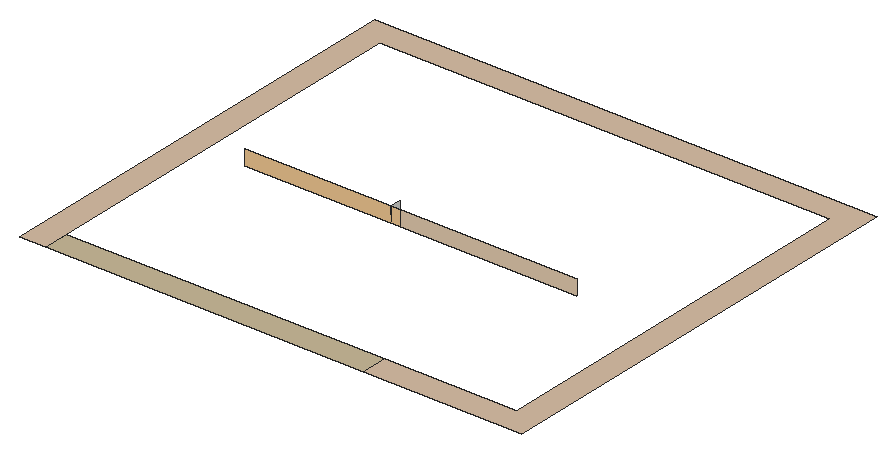
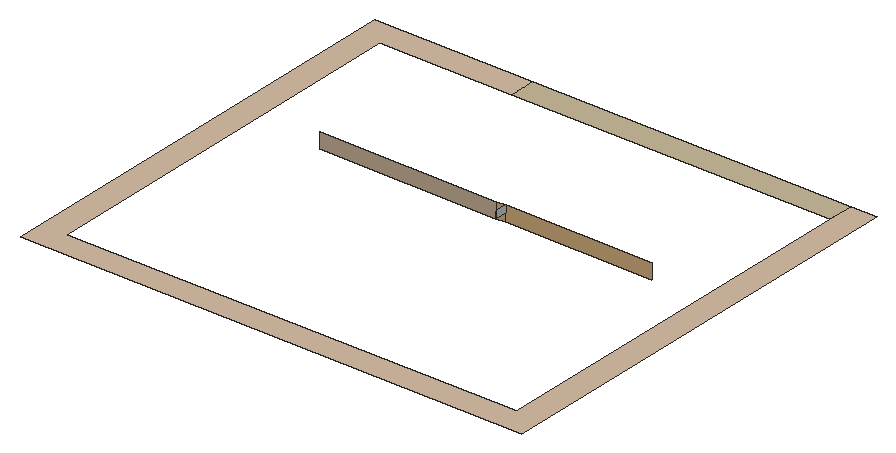
# SketchUp Ruby script. Lengths in inches.
U = 1.inch
M = Sketchup.active_model
def pt(a) = Geom::Point3d.new(a.map { |v| v * U })
def face(e, loops, mat)
  f = e.add_face(loops[0].map { |a| pt(a) })
  loops[1..].each { |l| e.add_face(l.map { |a| pt(a) }).erase! }
  f.material = f.back_material = mat if mat
  f
end
# faces: each face lists its corners as indices into pts; further lists are holes
def faces(e, pts, list, mat = nil) = list.each { |f| face(e, (f[0].is_a?(Array) ? f : [f]).map { |l| l.map { |i| pts[i] } }, mat) }
# xy, xz, yz: faces in a plane at the given z, y or x. An outline is a flat list of corners, or four numbers for a rectangle; further outlines are holes
def ring(l) = l.size == 4 ? [[l[0], l[1]], [l[2], l[1]], [l[2], l[3]], [l[0], l[3]]] : l.each_slice(2).to_a
def flat(e, list, mat, &to3) = list.each { |f| face(e, (f[0].is_a?(Array) ? f : [f]).map { |l| ring(l).map { |u, v| to3.(u, v) } }, mat) }
def xy(e, z, list, mat = nil) = flat(e, list, mat) { |x, y| [x, y, z] }
def xz(e, y, list, mat = nil) = flat(e, list, mat) { |x, z| [x, y, z] }
def yz(e, x, list, mat = nil) = flat(e, list, mat) { |y, z| [x, y, z] }
def lines(e, pts, list) = list.each { |a, b| e.add_line(pt(pts[a]), pt(pts[b])) }
# prism: a flat outline (further loops are holes) pulled along v
def prism(e, loops, v, mat = nil)
  f = face(e, loops, mat); d = Geom::Vector3d.new(v.map { |x| x * U })
  f.pushpull(f.normal.samedirection?(d) ? d.length : -d.length)
end
def box(e, o, s, mat = nil) = prism(e, [[o, [o[0] + s[0], o[1], o[2]], [o[0] + s[0], o[1] + s[1], o[2]], [o[0], o[1] + s[1], o[2]]]], [0, 0, s[2]], mat)
def at(x, y, z, deg = 0) = Geom::Transformation.translation(pt([x, y, z])) * Geom::Transformation.rotation(ORIGIN, Z_AXIS, deg.degrees)
def axes(o, x, y, z) = Geom::Transformation.new([*x, 0, *y, 0, *z, 0, *pt(o).to_a, 1])
def part(name) = M.definitions.add(name)
# library, detail: a bought-in or finely detailed component or shape, given as its bounding box
def library(name, o, s) = part(name).tap { |d| box(d.entities, o, s) }
def detail(e, o, s) = box(e.add_group.entities, o, s)
def put(e, d, t, mat = nil) = e.add_instance(d, t).tap { |i| i.material = mat if mat }
def group(e, t, mat = nil) = e.add_group.tap { |g| g.transformation = t; g.material = mat if mat }.entities
root = M.entities
M.materials.add("[0012_Bisque]").color = [234, 209, 180]
M.materials.add("[0036_BurlyWood]").color = [249, 207, 151]
M.materials.add("[Formica Laminate Light]").color = [213, 189, 164]
M.materials.add("[Quartz Light Brown]").color = [199, 184, 152]
xy(root,92.125,[[0,184.11,24.17,184.11,24.17,574.25,445.5,574.25,445.5,208.28,321.5,208.28,321.5,184.11,469.67,184.11,469.67,598.41,0,598.41]],"[Formica Laminate Light]")
xy(root,92.125,[[24.17,184.11,321.5,208.28]],"[Quartz Light Brown]")
xz(root,364.57,[[211.5,95.625,376.86,109.8125]],"[0012_Bisque]")
xz(root,364.57,[[65.97,95.625,202.72,109.8125],[202.72,95.625,211.5,109.8125]],"[0036_BurlyWood]")
yz(root,202.72,[[364.57,103.6875,374.1875,109.8125]])
